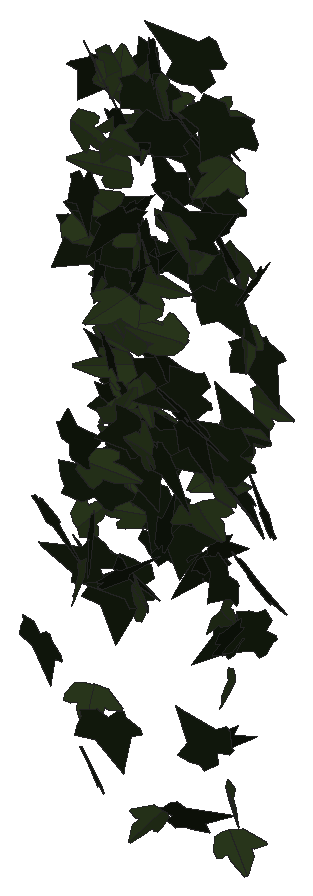
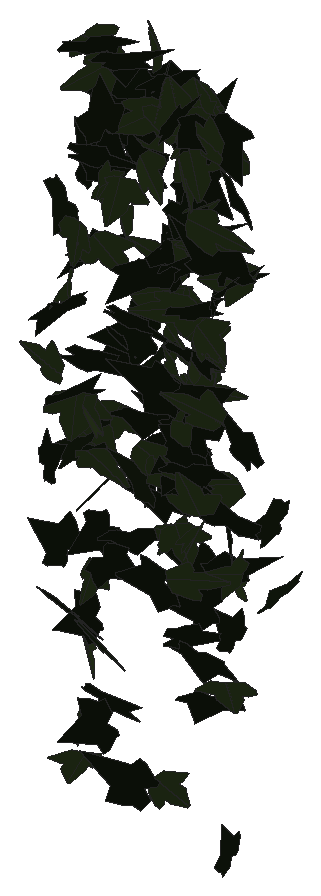
# SketchUp Ruby script. Lengths in inches.
U = 1.inch
M = Sketchup.active_model
def pt(a) = Geom::Point3d.new(a.map { |v| v * U })
def face(e, loops, mat)
  f = e.add_face(loops[0].map { |a| pt(a) })
  loops[1..].each { |l| e.add_face(l.map { |a| pt(a) }).erase! }
  f.material = f.back_material = mat if mat
  f
end
# faces: each face lists its corners as indices into pts; further lists are holes
def faces(e, pts, list, mat = nil) = list.each { |f| face(e, (f[0].is_a?(Array) ? f : [f]).map { |l| l.map { |i| pts[i] } }, mat) }
# xy, xz, yz: faces in a plane at the given z, y or x. An outline is a flat list of corners, or four numbers for a rectangle; further outlines are holes
def ring(l) = l.size == 4 ? [[l[0], l[1]], [l[2], l[1]], [l[2], l[3]], [l[0], l[3]]] : l.each_slice(2).to_a
def flat(e, list, mat, &to3) = list.each { |f| face(e, (f[0].is_a?(Array) ? f : [f]).map { |l| ring(l).map { |u, v| to3.(u, v) } }, mat) }
def xy(e, z, list, mat = nil) = flat(e, list, mat) { |x, y| [x, y, z] }
def xz(e, y, list, mat = nil) = flat(e, list, mat) { |x, z| [x, y, z] }
def yz(e, x, list, mat = nil) = flat(e, list, mat) { |y, z| [x, y, z] }
def lines(e, pts, list) = list.each { |a, b| e.add_line(pt(pts[a]), pt(pts[b])) }
# prism: a flat outline (further loops are holes) pulled along v
def prism(e, loops, v, mat = nil)
  f = face(e, loops, mat); d = Geom::Vector3d.new(v.map { |x| x * U })
  f.pushpull(f.normal.samedirection?(d) ? d.length : -d.length)
end
def box(e, o, s, mat = nil) = prism(e, [[o, [o[0] + s[0], o[1], o[2]], [o[0] + s[0], o[1] + s[1], o[2]], [o[0], o[1] + s[1], o[2]]]], [0, 0, s[2]], mat)
def at(x, y, z, deg = 0) = Geom::Transformation.translation(pt([x, y, z])) * Geom::Transformation.rotation(ORIGIN, Z_AXIS, deg.degrees)
def axes(o, x, y, z) = Geom::Transformation.new([*x, 0, *y, 0, *z, 0, *pt(o).to_a, 1])
def part(name) = M.definitions.add(name)
# library, detail: a bought-in or finely detailed component or shape, given as its bounding box
def library(name, o, s) = part(name).tap { |d| box(d.entities, o, s) }
def detail(e, o, s) = box(e.add_group.entities, o, s)
def put(e, d, t, mat = nil) = e.add_instance(d, t).tap { |i| i.material = mat if mat }
def group(e, t, mat = nil) = e.add_group.tap { |g| g.transformation = t; g.material = mat if mat }.entities
root = M.entities
M.materials.add("1026 AP 7946 SUNNY SIDE UP").color = [254, 231, 186]
M.materials.add("efeu1").color = [18, 25, 13]
M.materials.add("efeu2").color = [43, 57, 29]
c1 = part("ivyleaf_9")
p = [[1.54,2.16,1.25],[1.36,2.04,1.19],[-0.21,0.99,0.68],[-0.71,1.11,0.82],[-0.85,0.86,0.67],[-0.8,0.17,0.21],
  [-0.9,-0.01,0.1],[-0.67,-0.16,-0.02],[-0.08,-0.08,-0.05],[-0.03,-0.6,-0.4],[0.65,-0.88,-0.66],[0.83,-0.6,-0.49],
  [1.29,-0.42,-0.43],[1.8125,-0.07,-0.26],[1.21,0.44,0.15]]
faces(c1.entities,p,[[0,1,2,3,4,5,6,7,8,9,10,11,12,13,14]],"efeu1")
c2 = part("ivyleaf_10")
p = [[0,0.5,-0.03],[-0.0625,2.02,-0.43],[-0.19,2.01,-0.46],[-0.54,1.05,-0.29],[-0.52,0.625,-0.18],[-0.83,0.76,-0.28],
  [-1.16,0.64,-0.33],[-1.15,0.33,-0.24],[-0.77,-0.39,0.02],[-0.3,-0.51,0.16],[0.04,-0.48,0.23],[-0.02,2.01,-0.4375],
  [-0.06,2.01,-0.43],[0.04,-0.49,0.23],[0.67,-0.49,0.14],[1.38,0.36,-0.2],[1.375,0.51,-0.24],[0.81,0.65,-0.19],
  [0.62,0.59,-0.15],[0.6,1.09,-0.28],[0.5,1.23,-0.31]]
faces(c2.entities,p,[[0,1,2,3,4,5,6,7,8,9,10],[11,12,0,13,14,15,16,17,18,19,20]],"efeu2")
put(root,c1,axes([122.91,208.47,257],[0.052,-0.28438,0.12586],[0.02737,-0.12259,-0.29565],[0.48692,0.03726,0.00318]),"1026 AP 7946 SUNNY SIDE UP")
put(root,c2,axes([125.11,208.66,261.29],[-0.07327,0.06415,0.32052],[-0.45312,0.12294,-0.06994],[-0.20888,-0.28919,0.03929]),"1026 AP 7946 SUNNY SIDE UP")
put(root,c1,axes([124.98,209.11,261.03],[0.24105,-0.30269,0.00029],[-0.01967,-0.00858,-0.34925],[0.47555,0.15307,-0.01459]),"1026 AP 7946 SUNNY SIDE UP")
put(root,c2,axes([123.99,209.31,263.55],[0.26774,0.12233,-0.24182],[-0.27969,-0.15493,-0.21637],[-0.30954,0.2458,-0.01366]),"1026 AP 7946 SUNNY SIDE UP")
put(root,c2,axes([124.46,209.28,257.79],[-0.20932,0.2343,0.16689],[0.12927,-0.13807,0.27679],[0.4276,0.15644,-0.00198]),"1026 AP 7946 SUNNY SIDE UP")
put(root,c1,axes([122.34,209.28,258.96],[0.31027,-0.24501,0.02921],[0.00568,-0.03521,-0.3237],[0.38805,0.19642,-0.01861]),"1026 AP 7946 SUNNY SIDE UP")
put(root,c2,axes([126.24,209.37,266.87],[0.25108,0.15666,-0.24087],[-0.22786,-0.18587,-0.23047],[-0.38072,0.21456,-0.02092]),"1026 AP 7946 SUNNY SIDE UP")
put(root,c2,axes([122.98,209.52,257.77],[0.0898,-0.09039,0.30746],[0.22745,-0.26171,-0.11151],[0.43527,0.15541,-0.00516]),"1026 AP 7946 SUNNY SIDE UP")
put(root,c1,axes([123.66,209.375,255.2],[-0.16668,-0.22172,-0.15795],[0.1251,0.13026,-0.25204],[0.40381,-0.13188,0.01289]),"1026 AP 7946 SUNNY SIDE UP")
put(root,c2,axes([125.04,209.34,265.47],[-0.41934,0.12821,-0.12411],[0.14811,-0.08227,-0.30366],[-0.23457,-0.28115,0.03013]),"1026 AP 7946 SUNNY SIDE UP")
put(root,c1,axes([125.34,209.36,265.34],[-0.12609,0.04698,0.33267],[0.41033,-0.18997,0.0942],[0.30739,0.27285,0.01072]),"1026 AP 7946 SUNNY SIDE UP")
put(root,c2,axes([123.26,209.43,255.5625],[0.37744,0.15292,-0.04475],[-0.03871,-0.04354,-0.29248],[-0.24733,0.24018,-0.02251]),"1026 AP 7946 SUNNY SIDE UP")
put(root,c1,axes([123.88,209.54,265.09],[-0.0568,0.15892,-0.2765],[0.09327,-0.26269,-0.16943],[-0.48275,-0.06945,-0.0002]),"1026 AP 7946 SUNNY SIDE UP")
put(root,c1,axes([122.71,209.57,260.2],[-0.0129,0.06398,0.3174],[0.20133,-0.28045,0.06194],[0.45136,0.12693,-0.01856]),"1026 AP 7946 SUNNY SIDE UP")
put(root,c1,axes([124.875,209.55,261.74],[0.42428,-0.19278,0.13159],[0.14149,-0.09511,-0.34134],[0.336,0.28348,-0.02242]),"1026 AP 7946 SUNNY SIDE UP")
put(root,c1,axes([123.08,209.66,258.72],[-0.12143,0.00945,-0.31835],[0.42669,-0.15065,-0.07548],[-0.2331,-0.2807,0.02768]),"1026 AP 7946 SUNNY SIDE UP")
put(root,c2,axes([125.62,209.46,259.97],[-0.35612,-0.19944,-0.13793],[0.20042,0.05438,-0.30786],[0.31898,-0.25683,0.03944]),"1026 AP 7946 SUNNY SIDE UP")
put(root,c1,axes([125.25,209.625,261.34],[-0.10154,-0.0354,-0.30827],[0.47328,0.00128,-0.06711],[0.01373,-0.30592,0.03357]),"1026 AP 7946 SUNNY SIDE UP")
put(root,c1,axes([123.19,209.68,257.89],[-0.09932,0.03355,0.28792],[-0.42247,-0.09197,-0.05175],[0.131,-0.27117,0.05138]),"1026 AP 7946 SUNNY SIDE UP")
put(root,c1,axes([123.93,209.79,260.73],[-0.15151,-0.07845,0.27053],[-0.21853,-0.22647,-0.12335],[0.37221,-0.1649,0.0377]),"1026 AP 7946 SUNNY SIDE UP")
put(root,c2,axes([124.41,209.73,253.43],[-0.11177,-0.1962,0.19761],[-0.05362,-0.19144,-0.21463],[0.42934,-0.07499,0.02464]),"1026 AP 7946 SUNNY SIDE UP")
put(root,c1,axes([125.37,209.6875,262.03],[-0.43765,0.06222,0.12182],[-0.1907,-0.00489,-0.29233],[-0.08702,-0.30223,0.02797]),"1026 AP 7946 SUNNY SIDE UP")
put(root,c1,axes([122.8125,209.77,265.27],[-0.19975,-0.02229,-0.29041],[0.43793,-0.06255,-0.12463],[-0.07579,-0.30269,0.04529]),"1026 AP 7946 SUNNY SIDE UP")
put(root,c1,axes([126.1,209.83,261.04],[-0.48322,-0.02419,0.19037],[-0.28306,-0.0547,-0.31588],[0.07666,-0.35447,0.03362]),"1026 AP 7946 SUNNY SIDE UP")
put(root,c1,axes([125.79,209.96,258.5],[-0.09477,-0.18197,0.2249],[-0.07099,-0.21527,-0.19803],[0.44248,-0.07351,0.0164]),"1026 AP 7946 SUNNY SIDE UP")
put(root,c2,axes([124.36,209.94,267.55],[-0.05208,0.0401,-0.33706],[0.19669,-0.30295,-0.05304],[-0.47992,-0.12851,0.01484]),"1026 AP 7946 SUNNY SIDE UP")
put(root,c1,axes([125.69,209.99,264.8125],[0.04389,-0.1033,0.3622],[0.11595,-0.34441,-0.11211],[0.56532,0.07866,-0.00513]),"1026 AP 7946 SUNNY SIDE UP")
put(root,c1,axes([123.48,209.6,257.77],[0.08996,0.27049,-0.08686],[0.00946,0.0864,0.28508],[0.44612,-0.05638,0.01147]),"1026 AP 7946 SUNNY SIDE UP")
put(root,c2,axes([124.65,209.91,262.76],[0.07173,0.11145,0.29295],[-0.24872,-0.23659,0.12055],[0.40975,-0.16313,0.02189]),"1026 AP 7946 SUNNY SIDE UP")
put(root,c1,axes([124.67,209.61,258.97],[-0.05455,-0.05036,0.29587],[0.17106,0.26641,0.06316],[-0.42585,0.11347,-0.01253]),"1026 AP 7946 SUNNY SIDE UP")
put(root,c2,axes([123.75,209.98,264.34],[-0.03909,0.05404,0.34396],[0.4317,-0.19178,0.05196],[0.30979,0.27406,-0.02902]),"1026 AP 7946 SUNNY SIDE UP")
put(root,c2,axes([123.56,209.81,260.93],[-0.22227,-0.25781,0.06645],[0.0304,0.06455,0.30294],[-0.41733,0.14201,-0.01332]),"1026 AP 7946 SUNNY SIDE UP")
put(root,c2,axes([123.88,209.98,261.53],[0.27376,-0.0537,0.27756],[0.36366,-0.14416,-0.1842],[0.23401,0.28685,-0.03845]),"1026 AP 7946 SUNNY SIDE UP")
put(root,c2,axes([123.59,209.86,262.43],[-0.52307,0.01326,0.07434],[0.11434,0.01787,0.34244],[0.01439,0.33991,-0.0189]),"1026 AP 7946 SUNNY SIDE UP")
put(root,c1,axes([123.71,209.99,264.1875],[-0.22895,-0.27318,-0.08176],[-0.08148,-0.06042,0.31809],[-0.43914,0.15364,-0.0164]),"1026 AP 7946 SUNNY SIDE UP")
put(root,c2,axes([123.7,210.02,264.51],[-0.03307,0.19622,0.24004],[-0.06831,-0.232,0.19682],[0.47273,-0.0198,0.04523]),"1026 AP 7946 SUNNY SIDE UP")
put(root,c1,axes([124.36,209.73,266.625],[-0.046,0.01472,0.33994],[0.50149,0.08711,0.02564],[-0.1346,0.31952,-0.02064]),"1026 AP 7946 SUNNY SIDE UP")
put(root,c1,axes([123.95,210.15,264.39],[0.14433,-0.15168,-0.30105],[0.35771,-0.18888,0.17403],[-0.3726,-0.24009,0.05045]),"1026 AP 7946 SUNNY SIDE UP")
put(root,c2,axes([122.55,210.03,266.17],[-0.064,-0.00808,-0.31576],[0.37401,-0.19587,-0.02837],[-0.30412,-0.23918,0.03156]),"1026 AP 7946 SUNNY SIDE UP")
put(root,c2,axes([126,209.875,253.46],[0.2614,0.23137,0.06627],[0.08046,0.04068,-0.29272],[-0.36838,0.17307,-0.01691]),"1026 AP 7946 SUNNY SIDE UP")
put(root,c1,axes([123.27,209.82,262.27],[0.24098,-0.08027,-0.27404],[-0.40486,0.07179,-0.17502],[0.16239,0.29808,-0.02967]),"1026 AP 7946 SUNNY SIDE UP")
put(root,c2,axes([125.92,209.89,254.31],[-0.20554,0.25247,0.02016],[-0.03257,0.00967,-0.29248],[-0.39667,-0.13162,0.01357]),"1026 AP 7946 SUNNY SIDE UP")
put(root,c1,axes([125.66,210.16,267.33],[-0.33724,-0.28026,0.0214],[0.00468,-0.03039,-0.36311],[0.44206,-0.21348,0.02017]),"1026 AP 7946 SUNNY SIDE UP")
put(root,c2,axes([122.92,209.89,259.74],[-0.12256,-0.07961,-0.29708],[0.44583,0.07396,-0.09971],[0.14787,-0.28897,0.05439]),"1026 AP 7946 SUNNY SIDE UP")
put(root,c1,axes([125.29,210.06,264.97],[0.24037,0.16099,0.22499],[-0.26361,-0.13971,0.22712],[0.33396,-0.22615,0.01734]),"1026 AP 7946 SUNNY SIDE UP")
put(root,c2,axes([123.46,209.84,266.3],[-0.14957,-0.18525,-0.26181],[0.21552,0.21333,-0.21269],[0.44359,-0.16611,0.01505]),"1026 AP 7946 SUNNY SIDE UP")
put(root,c2,axes([123.91,209.99,263.6],[-0.14265,0.00212,0.33785],[0.5095,0.05298,0.0923],[-0.07941,0.3361,-0.01467]),"1026 AP 7946 SUNNY SIDE UP")
put(root,c1,axes([122.54,210.3,263.82],[-0.21097,-0.20328,0.23571],[-0.14504,-0.21266,-0.25035],[0.4603,-0.16018,0.02915]),"1026 AP 7946 SUNNY SIDE UP")
put(root,c2,axes([123.76,209.95,262.81],[-0.14829,-0.07559,-0.32869],[0.49688,0.06596,-0.11209],[0.13505,-0.32568,0.0515]),"1026 AP 7946 SUNNY SIDE UP")
put(root,c1,axes([124.65,209.99,253.41],[0.32203,0.14038,-0.14692],[0.1625,0.10187,0.25537],[0.27049,-0.22833,0.0215]),"1026 AP 7946 SUNNY SIDE UP")
put(root,c1,axes([122.83,210.27,263.69],[0.00002,-0.03159,-0.30827],[0.35085,-0.20048,0.02066],[-0.317,-0.2219,0.02284]),"1026 AP 7946 SUNNY SIDE UP")
put(root,c2,axes([123.25,210.25,261.63],[0.10702,0.01212,-0.30199],[-0.41105,-0.13426,-0.06901],[-0.20967,0.2694,-0.01884]),"1026 AP 7946 SUNNY SIDE UP")
put(root,c1,axes([123.61,210.17,264.91],[-0.1542,0.22825,-0.20385],[0.10241,-0.18856,-0.25676],[-0.46519,-0.11717,0.01105]),"1026 AP 7946 SUNNY SIDE UP")
put(root,c1,axes([122.88,210.01,259.08],[-0.44993,0.10726,0.17848],[0.266,-0.03956,0.31394],[0.17714,0.33184,-0.01809]),"1026 AP 7946 SUNNY SIDE UP")
put(root,c2,axes([123.91,210.25,266.48],[0.28869,-0.21245,0.11387],[0.09165,-0.09701,-0.28924],[0.36614,0.19179,-0.01738]),"1026 AP 7946 SUNNY SIDE UP")
put(root,c2,axes([123.43,210.38,260.94],[-0.12557,-0.10062,0.30724],[-0.04281,-0.30489,-0.11505],[0.49392,-0.052,0.06814]),"1026 AP 7946 SUNNY SIDE UP")
put(root,c1,axes([124.42,210.28,266.8],[0.28611,-0.19868,0.18737],[0.16795,-0.14975,-0.27777],[0.39013,0.21018,-0.01783]),"1026 AP 7946 SUNNY SIDE UP")
put(root,c1,axes([125.42,210.1,254.89],[-0.40671,-0.03312,-0.13047],[-0.20103,0.0057,0.2679],[-0.04281,0.28785,-0.0186]),"1026 AP 7946 SUNNY SIDE UP")
put(root,c1,axes([124.28,210.3,259.31],[-0.42409,-0.09613,-0.13684],[0.2111,0.0155,-0.2935],[0.1468,-0.3,0.02675]),"1026 AP 7946 SUNNY SIDE UP")
put(root,c1,axes([124.96,210.28,266.54],[-0.34401,-0.13061,-0.21179],[0.30945,0.06633,-0.25972],[0.22395,-0.29227,0.03356]),"1026 AP 7946 SUNNY SIDE UP")
put(root,c1,axes([123.92,209.89,263.68],[0.07492,0.11386,0.35364],[0.29074,0.28914,-0.12379],[-0.48762,0.18989,-0.01947]),"1026 AP 7946 SUNNY SIDE UP")
put(root,c1,axes([123.84,210.23,267.32],[-0.02141,-0.28633,-0.15882],[0.02391,0.15194,-0.29434],[0.50957,-0.01916,0.00714]),"1026 AP 7946 SUNNY SIDE UP")
put(root,c1,axes([123.16,210.27,260.74],[0.17767,-0.0418,0.35307],[0.41967,-0.21858,-0.11931],[0.34498,0.28742,-0.03669]),"1026 AP 7946 SUNNY SIDE UP")
put(root,c1,axes([124.38,210.31,260.76],[-0.2791,-0.1935,-0.12378],[0.14745,0.07521,-0.26952],[0.32539,-0.20006,0.01597]),"1026 AP 7946 SUNNY SIDE UP")
put(root,c1,axes([123.15,210.38,266.07],[0.10793,-0.06925,0.31081],[0.2447,-0.25988,-0.09932],[0.42145,0.16862,-0.02193]),"1026 AP 7946 SUNNY SIDE UP")
put(root,c1,axes([122.91,210.3,266.9],[0.13024,-0.24233,0.15667],[-0.02573,0.15547,0.26294],[-0.45028,-0.07898,0.03029]),"1026 AP 7946 SUNNY SIDE UP")
put(root,c2,axes([122.41,210.04,263.89],[0.11533,0.02835,-0.35889],[0.32902,0.28176,0.07063],[0.44054,-0.21786,0.04121]),"1026 AP 7946 SUNNY SIDE UP")
put(root,c1,axes([123.69,210.5,263.77],[-0.21136,-0.07678,0.25431],[-0.27682,-0.17723,-0.1563],[0.29858,-0.21866,0.03511]),"1026 AP 7946 SUNNY SIDE UP")
put(root,c2,axes([124.61,210.44,264.28],[-0.17243,0.11018,0.29684],[0.37701,-0.16093,0.1568],[0.30375,0.26228,-0.02611]),"1026 AP 7946 SUNNY SIDE UP")
put(root,c2,axes([123.07,210.25,267.32],[0.23276,-0.19203,-0.18197],[-0.19768,0.12403,-0.24827],[0.35817,0.19325,-0.01877]),"1026 AP 7946 SUNNY SIDE UP")
put(root,c1,axes([124.46,210.18,265.42],[0.09893,-0.02285,0.30608],[-0.21501,0.26773,0.05258],[-0.41653,-0.14362,0.04555]),"1026 AP 7946 SUNNY SIDE UP")
put(root,c1,axes([123.45,210.39,259.91],[-0.23824,-0.12909,-0.25058],[0.32261,0.13099,-0.20313],[0.28726,-0.25417,0.02031]),"1026 AP 7946 SUNNY SIDE UP")
put(root,c1,axes([122.85,210.4,257.66],[0.34462,-0.13702,0.14732],[0.16949,-0.09778,-0.26584],[0.26231,0.2432,-0.02178]),"1026 AP 7946 SUNNY SIDE UP")
put(root,c1,axes([123.47,210.375,263.01],[-0.32852,-0.2011,0.01594],[-0.00288,0.02581,0.29819],[-0.31728,0.20799,-0.01922]),"1026 AP 7946 SUNNY SIDE UP")
put(root,c1,axes([123.46,210.24,260.41],[0.36257,0.19521,-0.02861],[-0.01232,-0.03533,-0.31064],[-0.31005,0.22969,-0.02111]),"1026 AP 7946 SUNNY SIDE UP")
put(root,c1,axes([125.27,210.35,263.6875],[0.09727,-0.25097,-0.20992],[-0.00521,0.20553,-0.26246],[0.50689,0.05027,0.03758]),"1026 AP 7946 SUNNY SIDE UP")
put(root,c2,axes([122.68,210.37,264.51],[0.16797,0.05972,0.30113],[0.45255,0.05979,-0.12073],[-0.12157,0.30509,-0.03336]),"1026 AP 7946 SUNNY SIDE UP")
put(root,c1,axes([125.16,210.44,260.05],[0.3367,-0.18479,0.05762],[0.0483,-0.05144,-0.29105],[0.3002,0.21553,-0.0178]),"1026 AP 7946 SUNNY SIDE UP")
put(root,c2,axes([123.12,210.34,267.1],[0.47269,0.03147,-0.01146],[0.01275,0.03058,0.31007],[0.05101,-0.29927,0.02869]),"1026 AP 7946 SUNNY SIDE UP")
put(root,c1,axes([126.12,210.14,264.13],[0.03884,0.20877,0.25476],[0.05759,0.24342,-0.21509],[-0.50419,0.04389,-0.00494]),"1026 AP 7946 SUNNY SIDE UP")
put(root,c1,axes([122.21,210.59,257.38],[0.08659,-0.14828,0.227],[0.11244,-0.20934,-0.16414],[0.40334,0.09019,-0.00298]),"1026 AP 7946 SUNNY SIDE UP")
put(root,c2,axes([122.46,210.19,258.32],[0.07968,0.08195,-0.30007],[0.1938,0.26465,0.10019],[0.4353,-0.13282,0.01032]),"1026 AP 7946 SUNNY SIDE UP")
put(root,c1,axes([123.53,210.41,261.27],[0.10279,-0.00241,0.3529],[-0.47817,0.16018,0.06188],[-0.24804,-0.30979,0.02696]),"1026 AP 7946 SUNNY SIDE UP")
put(root,c2,axes([125.13,210.47,259.89],[-0.25253,0.02095,0.29491],[0.44951,-0.01624,0.16642],[0.03842,0.32774,-0.00868]),"1026 AP 7946 SUNNY SIDE UP")
put(root,c1,axes([122.53,210.4375,264.13],[-0.15944,0.07884,0.34056],[0.43808,-0.17746,0.13078],[0.30483,0.29627,-0.00981]),"1026 AP 7946 SUNNY SIDE UP")
put(root,c2,axes([125.53,210.38,256.125],[0.12271,-0.25654,-0.15203],[-0.08392,0.13639,-0.27525],[0.45658,0.09401,-0.00973]),"1026 AP 7946 SUNNY SIDE UP")
put(root,c1,axes([123.34,210.23,260.49],[0.23601,0.1985,0.17893],[0.17938,0.12988,-0.25539],[-0.37265,0.18824,-0.00962]),"1026 AP 7946 SUNNY SIDE UP")
put(root,c1,axes([125.43,210.63,259.91],[0.19218,-0.27727,0.10306],[0.0614,-0.09383,-0.31271],[0.46027,0.12829,-0.00132]),"1026 AP 7946 SUNNY SIDE UP")
put(root,c1,axes([125.42,210.6,265.48],[-0.33838,0.01545,0.21253],[-0.32424,-0.03849,-0.21894],[0.02453,-0.29556,0.03786]),"1026 AP 7946 SUNNY SIDE UP")
put(root,c2,axes([125.35,210.37,257.48],[-0.05713,-0.21763,-0.2111],[0.06784,0.19918,-0.22602],[0.46376,-0.05595,0.00706]),"1026 AP 7946 SUNNY SIDE UP")
put(root,c1,axes([125.16,210.38,263.58],[-0.22903,-0.1007,0.23809],[0.26306,0.16193,0.18181],[-0.29763,0.22061,-0.02252]),"1026 AP 7946 SUNNY SIDE UP")
put(root,c2,axes([123.1,210.35,262.45],[-0.02824,0.00349,-0.32012],[-0.3217,0.23418,0.01626],[0.36784,0.20507,-0.01036]),"1026 AP 7946 SUNNY SIDE UP")
put(root,c1,axes([122.1875,210.7,253.28],[0.21355,-0.09955,-0.22319],[0.30447,-0.0983,0.17146],[-0.21735,-0.23552,0.02091]),"1026 AP 7946 SUNNY SIDE UP")
put(root,c2,axes([123.78,210.72,260.08],[0.01394,-0.02961,-0.29847],[-0.24025,-0.24703,0.01976],[-0.38953,0.1513,-0.02286]),"1026 AP 7946 SUNNY SIDE UP")
put(root,c2,axes([125.2,210.31,267.07],[-0.0734,-0.10696,-0.36055],[0.27657,0.30214,-0.11773],[0.50358,-0.18153,0.01211]),"1026 AP 7946 SUNNY SIDE UP")
put(root,c2,axes([123.37,210.6,266.8],[-0.33853,-0.29267,0.01638],[-0.00147,0.02247,0.37415],[-0.46102,0.21484,-0.01322]),"1026 AP 7946 SUNNY SIDE UP")
put(root,c1,axes([124.3,210.72,258.7],[-0.25911,-0.27291,-0.05587],[0.07205,0.03374,-0.32748],[0.43107,-0.16968,0.02116]),"1026 AP 7946 SUNNY SIDE UP")
put(root,c2,axes([125.72,210.67,262.92],[-0.01224,0.26343,-0.17825],[0.0019,-0.17455,-0.27251],[-0.49687,-0.00715,0.00335]),"1026 AP 7946 SUNNY SIDE UP")
put(root,c2,axes([122.92,210.81,262.39],[-0.03781,0.06951,0.3361],[0.29569,-0.26686,0.07138],[0.43248,0.18853,-0.01942]),"1026 AP 7946 SUNNY SIDE UP")
put(root,c2,axes([123.05,210.63,266.18],[-0.18625,-0.30712,0.01585],[0.00704,-0.02008,-0.33902],[0.48362,-0.11798,0.01104]),"1026 AP 7946 SUNNY SIDE UP")
put(root,c1,axes([122.86,210.7,256.89],[-0.36375,-0.10566,-0.17942],[0.26437,0.04816,-0.26078],[0.17942,-0.28517,0.02049]),"1026 AP 7946 SUNNY SIDE UP")
put(root,c1,axes([124.78,210.79,258.09],[-0.04412,0.06289,-0.29434],[0.11824,-0.2762,-0.07177],[-0.44513,-0.0796,0.01011]),"1026 AP 7946 SUNNY SIDE UP")
put(root,c1,axes([123.26,210.8,257.09],[-0.24258,-0.0543,0.24458],[-0.32723,-0.11728,-0.16742],[0.19982,-0.25798,0.02275]),"1026 AP 7946 SUNNY SIDE UP")
put(root,c2,axes([122.68,210.77,263.08],[-0.03196,-0.29088,0.14827],[-0.00355,-0.14573,-0.30116],[0.51145,-0.01919,0.00718]),"1026 AP 7946 SUNNY SIDE UP")
put(root,c1,axes([123.55,210.68,261.63],[0.28587,-0.02169,-0.26873],[0.3937,0.10653,0.17136],[0.11935,-0.29948,0.07843]),"1026 AP 7946 SUNNY SIDE UP")
put(root,c2,axes([123.85,210.58,266.8],[-0.28439,-0.12096,-0.29106],[0.39757,0.1264,-0.2223],[0.27298,-0.31011,0.02053]),"1026 AP 7946 SUNNY SIDE UP")
put(root,c1,axes([122.59,210.7,267.06],[0.17822,0.19933,-0.2491],[-0.16457,-0.21956,-0.23719],[-0.46591,0.15381,-0.01151]),"1026 AP 7946 SUNNY SIDE UP")
put(root,c1,axes([125.56,210.87,258.04],[0.17673,-0.18338,0.25133],[0.19204,-0.21245,-0.22277],[0.44124,0.16592,-0.00371]),"1026 AP 7946 SUNNY SIDE UP")
put(root,c2,axes([124.92,210.78,264.03],[-0.332,-0.12775,0.18307],[-0.20034,-0.13023,-0.25214],[0.28094,-0.24384,0.03653]),"1026 AP 7946 SUNNY SIDE UP")
put(root,c1,axes([125.05,210.46,254.69],[0.17331,0.15931,0.24136],[0.23862,0.17794,-0.19792],[-0.3748,0.18695,-0.01441]),"1026 AP 7946 SUNNY SIDE UP")
put(root,c1,axes([125.01,210.46,258.45],[-0.05125,0.10112,-0.29267],[-0.14722,0.26884,0.11099],[0.45162,0.09911,0.00297]),"1026 AP 7946 SUNNY SIDE UP")
put(root,c1,axes([126.19,210.61,259.31],[0.02732,-0.13977,0.27261],[-0.0627,0.26242,0.14659],[-0.46748,-0.04337,-0.00373]),"1026 AP 7946 SUNNY SIDE UP")
put(root,c2,axes([122.8,210.75,265.08],[-0.07413,0.02608,0.34816],[-0.51075,-0.10047,-0.0393],[0.1515,-0.32595,0.03787]),"1026 AP 7946 SUNNY SIDE UP")
put(root,c1,axes([123.04,210.83,262.66],[-0.40303,-0.07166,-0.09348],[0.14726,-0.00093,-0.273],[0.10577,-0.27176,0.02388]),"1026 AP 7946 SUNNY SIDE UP")
put(root,c1,axes([123.62,210.6,267.67],[0.19135,-0.11047,-0.26286],[-0.33226,0.14323,-0.16728],[0.28276,0.24306,-0.01868]),"1026 AP 7946 SUNNY SIDE UP")
put(root,c2,axes([124.99,210.78,259.9375],[0.38611,0.014,-0.16687],[-0.25114,-0.03485,-0.25261],[-0.04846,0.29214,-0.0204]),"1026 AP 7946 SUNNY SIDE UP")
put(root,c1,axes([125.74,210.78,262.58],[0.04212,-0.308,-0.1321],[-0.0252,0.12555,-0.31773],[0.52294,0.03086,-0.00467]),"1026 AP 7946 SUNNY SIDE UP")
put(root,c1,axes([122.96,210.86,260.47],[-0.31547,-0.2048,-0.06873],[0.08928,0.03602,-0.29474],[0.32612,-0.20797,0.0142]),"1026 AP 7946 SUNNY SIDE UP")
put(root,c2,axes([123.94,210.76,260.36],[-0.18637,0.01852,0.27413],[-0.40942,-0.07072,-0.11487],[0.09028,-0.28248,0.04497]),"1026 AP 7946 SUNNY SIDE UP")
put(root,c2,axes([125.45,210.75,260.81],[-0.41722,-0.18919,-0.02406],[0.05183,-0.00797,-0.33473],[0.29502,-0.26615,0.02478]),"1026 AP 7946 SUNNY SIDE UP")
put(root,c1,axes([124.03,210.64,259.69],[-0.03844,0.28972,0.03445],[0.0015,-0.03183,0.29934],[0.45829,0.02441,0.00191]),"1026 AP 7946 SUNNY SIDE UP")
put(root,c1,axes([125.67,210.78,260.77],[-0.31061,-0.2475,0.09271],[0.07342,0.07958,0.32644],[-0.40831,0.20259,-0.01183]),"1026 AP 7946 SUNNY SIDE UP")
put(root,c2,axes([122.93,210.71,259.21],[-0.01905,0.28435,0.04801],[-0.00547,0.04488,-0.29294],[-0.45265,-0.01251,0.00152]),"1026 AP 7946 SUNNY SIDE UP")
put(root,c2,axes([122.85,210.8,259.76],[-0.35524,-0.11289,0.09669],[0.11879,0.05965,0.25984],[-0.19868,0.23751,-0.01752]),"1026 AP 7946 SUNNY SIDE UP")
put(root,c1,axes([125.21,210.57,256.72],[0.09434,0.12841,0.26946],[0.24132,0.21221,-0.14275],[-0.38825,0.1631,-0.02326]),"1026 AP 7946 SUNNY SIDE UP")
put(root,c1,axes([124.64,211,266.45],[0.41552,-0.18056,-0.12835],[0.19686,-0.03411,0.32698],[-0.28214,-0.28972,0.03912]),"1026 AP 7946 SUNNY SIDE UP")
put(root,c2,axes([123.8125,210.91,265.94],[0.0319,-0.3245,0.07168],[0.00153,-0.0715,-0.33535],[0.52245,0.02002,-0.0034]),"1026 AP 7946 SUNNY SIDE UP")
put(root,c2,axes([123.09,210.81,266.08],[0.12147,-0.30499,-0.07827],[-0.0179,0.07369,-0.32361],[0.49324,0.07779,0.00753]),"1026 AP 7946 SUNNY SIDE UP")
put(root,c1,axes([124.6,210.89,267.65],[-0.33321,-0.24415,-0.07182],[-0.09884,-0.03568,0.33196],[-0.38621,0.21978,-0.02299]),"1026 AP 7946 SUNNY SIDE UP")
put(root,c1,axes([123.5,210.87,258.1],[0.06751,-0.03022,-0.30383],[0.44709,0.088,0.03389],[0.13109,-0.28457,0.0409]),"1026 AP 7946 SUNNY SIDE UP")
put(root,c2,axes([123.05,210.97,258.34],[0.01237,0.06047,0.30053],[-0.29333,-0.2261,0.0522],[0.36458,-0.18396,0.0318]),"1026 AP 7946 SUNNY SIDE UP")
put(root,c2,axes([124.97,210.98,260.89],[0.16999,-0.23179,0.14754],[0.07892,-0.13594,-0.26407],[0.42221,0.11874,-0.01005]),"1026 AP 7946 SUNNY SIDE UP")
put(root,c1,axes([125.83,210.91,257.03],[-0.4448,0.08972,-0.00582],[-0.00445,-0.02921,-0.30446],[-0.14134,-0.28143,0.02791]),"1026 AP 7946 SUNNY SIDE UP")
put(root,c2,axes([123.13,210.91,259.18],[-0.25408,-0.2292,0.06371],[-0.0359,-0.06103,-0.28878],[0.37209,-0.16239,0.01564]),"1026 AP 7946 SUNNY SIDE UP")
put(root,c2,axes([124.61,211.0625,265.4],[0.00998,0.03726,-0.28455],[-0.08793,-0.2707,-0.04049],[-0.42966,0.05627,0.00168]),"1026 AP 7946 SUNNY SIDE UP")
put(root,c2,axes([122.35,210.94,266.84],[-0.07664,0.02556,0.33441],[0.50478,-0.05022,0.05346],[0.08423,0.32423,-0.01613]),"1026 AP 7946 SUNNY SIDE UP")
put(root,c1,axes([123.85,210.8,263.93],[-0.01959,-0.18832,-0.27099],[0.05585,0.25978,-0.1926],[0.50424,-0.03609,0.0108]),"1026 AP 7946 SUNNY SIDE UP")
put(root,c1,axes([125.15,210.93,256.72],[-0.40224,0.1236,-0.07822],[0.08712,-0.06051,-0.29147],[-0.21142,-0.26009,0.0287]),"1026 AP 7946 SUNNY SIDE UP")
put(root,c2,axes([125.74,210.94,261.44],[-0.07662,0.02419,0.30088],[0.45539,-0.04036,0.05301],[0.06901,0.29319,-0.01576]),"1026 AP 7946 SUNNY SIDE UP")
put(root,c2,axes([123.38,210.6875,259],[0.0986,0.14092,-0.25224],[0.10808,0.2365,0.15923],[0.43199,-0.09133,0.01773]),"1026 AP 7946 SUNNY SIDE UP")
put(root,c2,axes([122.52,210.83,261.6],[-0.15178,-0.01248,0.30225],[0.41724,0.12876,0.09631],[-0.19806,0.28082,-0.02873]),"1026 AP 7946 SUNNY SIDE UP")
put(root,c2,axes([124.44,210.87,265.31],[-0.25584,-0.26558,-0.10397],[0.11033,0.07335,-0.31974],[0.43203,-0.176,0.02008]),"1026 AP 7946 SUNNY SIDE UP")
put(root,c1,axes([123.18,211.18,266.95],[-0.09572,-0.04576,0.32857],[-0.23717,-0.28308,-0.07309],[0.44816,-0.15958,0.0315]),"1026 AP 7946 SUNNY SIDE UP")
put(root,c2,axes([125.32,210.89,264.19],[-0.39442,0.17408,0.03413],[-0.07039,-0.00844,-0.31283],[-0.2693,-0.25275,0.03177]),"1026 AP 7946 SUNNY SIDE UP")
